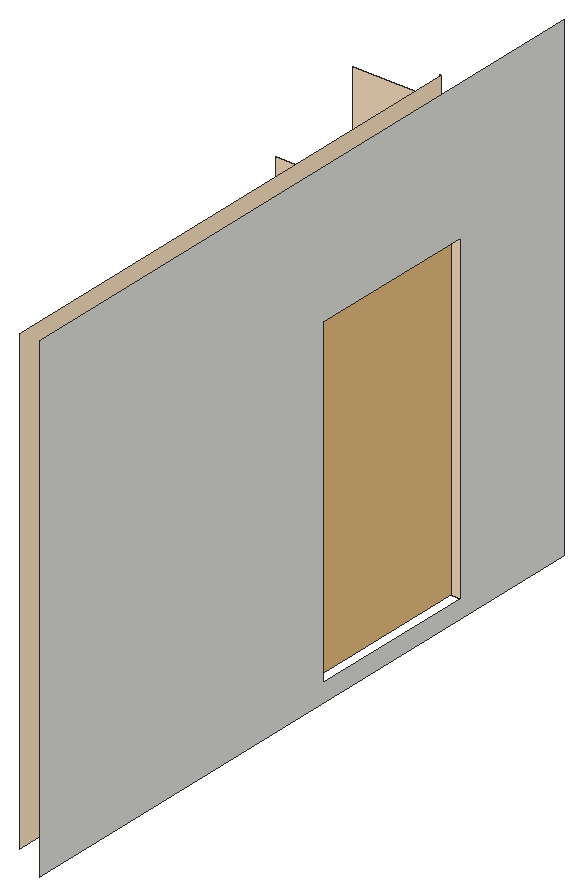
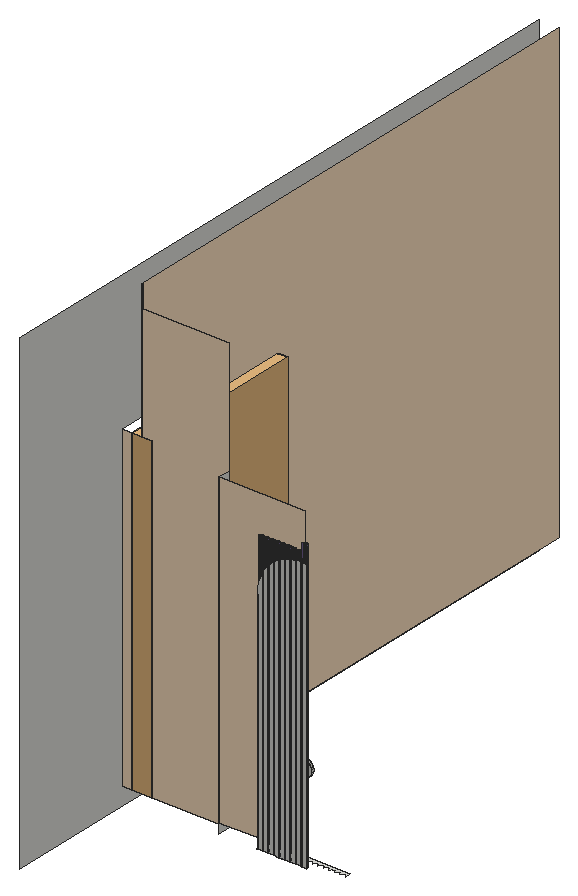
# SketchUp Ruby script. Lengths in inches.
U = 1.inch
M = Sketchup.active_model
def pt(a) = Geom::Point3d.new(a.map { |v| v * U })
def face(e, loops, mat)
  f = e.add_face(loops[0].map { |a| pt(a) })
  loops[1..].each { |l| e.add_face(l.map { |a| pt(a) }).erase! }
  f.material = f.back_material = mat if mat
  f
end
# faces: each face lists its corners as indices into pts; further lists are holes
def faces(e, pts, list, mat = nil) = list.each { |f| face(e, (f[0].is_a?(Array) ? f : [f]).map { |l| l.map { |i| pts[i] } }, mat) }
# xy, xz, yz: faces in a plane at the given z, y or x. An outline is a flat list of corners, or four numbers for a rectangle; further outlines are holes
def ring(l) = l.size == 4 ? [[l[0], l[1]], [l[2], l[1]], [l[2], l[3]], [l[0], l[3]]] : l.each_slice(2).to_a
def flat(e, list, mat, &to3) = list.each { |f| face(e, (f[0].is_a?(Array) ? f : [f]).map { |l| ring(l).map { |u, v| to3.(u, v) } }, mat) }
def xy(e, z, list, mat = nil) = flat(e, list, mat) { |x, y| [x, y, z] }
def xz(e, y, list, mat = nil) = flat(e, list, mat) { |x, z| [x, y, z] }
def yz(e, x, list, mat = nil) = flat(e, list, mat) { |y, z| [x, y, z] }
def lines(e, pts, list) = list.each { |a, b| e.add_line(pt(pts[a]), pt(pts[b])) }
# prism: a flat outline (further loops are holes) pulled along v
def prism(e, loops, v, mat = nil)
  f = face(e, loops, mat); d = Geom::Vector3d.new(v.map { |x| x * U })
  f.pushpull(f.normal.samedirection?(d) ? d.length : -d.length)
end
def box(e, o, s, mat = nil) = prism(e, [[o, [o[0] + s[0], o[1], o[2]], [o[0] + s[0], o[1] + s[1], o[2]], [o[0], o[1] + s[1], o[2]]]], [0, 0, s[2]], mat)
def at(x, y, z, deg = 0) = Geom::Transformation.translation(pt([x, y, z])) * Geom::Transformation.rotation(ORIGIN, Z_AXIS, deg.degrees)
def axes(o, x, y, z) = Geom::Transformation.new([*x, 0, *y, 0, *z, 0, *pt(o).to_a, 1])
def part(name) = M.definitions.add(name)
# library, detail: a bought-in or finely detailed component or shape, given as its bounding box
def library(name, o, s) = part(name).tap { |d| box(d.entities, o, s) }
def detail(e, o, s) = box(e.add_group.entities, o, s)
def put(e, d, t, mat = nil) = e.add_instance(d, t).tap { |i| i.material = mat if mat }
def group(e, t, mat = nil) = e.add_group.tap { |g| g.transformation = t; g.material = mat if mat }.entities
root = M.entities
M.materials.add("[0012_Bisque]").color = [255, 228, 196]
M.materials.add("[Color I01]").color = [116, 98, 147]
c1 = part("Group\#9")
xz(c1.entities,0,[[0.27,0,0.25,0.59,0.18,0.57,0.11,0.53,0.06,0.47,0.02,0.4,0,0.33,0,0.25,0.02,0.18,0.07,0.11,0.125,0.06,0.19,0.02],[0.35,0,0.42,0.02,0.49,0.07,0.54,0.125,0.58,0.19,0.6,0.27,0.59,0.35,0.57,0.42,0.53,0.49,0.47,0.54,0.4,0.58,0.33,0.6]])
xz(c1.entities,0.0625,[[0.27,0,0.35,0,0.33,0.6,0.25,0.59]])
yz(c1.entities,0,[[0,0.25,0.0625,0.33]])
p = [[0.125,0.0625,0.06],[0.19,0.0625,0.02],[0.19,0,0.02],[0.125,0,0.06],[0.27,0.0625,0],[0.27,0,0],
  [0.33,0.0625,0.6],[0.35,0.0625,0],[0.35,0,0],[0.33,0,0.6],[0.42,0.0625,0.02],[0.42,0,0.02],
  [0.25,0.0625,0.59],[0.25,0,0.59],[0.49,0.0625,0.07],[0.49,0,0.07],[0.02,0.0625,0.18],[0.07,0.0625,0.11],
  [0.07,0,0.11],[0.02,0,0.18],[0.54,0.0625,0.125],[0.54,0,0.125],[0.58,0.0625,0.19],[0.58,0,0.19],
  [0,0.0625,0.25],[0,0,0.25],[0.6,0.0625,0.27],[0.6,0,0.27],[0.02,0.0625,0.4],[0,0.0625,0.33],
  [0,0,0.33],[0.02,0,0.4],[0.59,0.0625,0.35],[0.57,0.0625,0.42],[0.57,0,0.42],[0.59,0,0.35],
  [0.06,0.0625,0.47],[0.06,0,0.47],[0.53,0.0625,0.49],[0.53,0,0.49],[0.18,0.0625,0.57],[0.11,0.0625,0.53],
  [0.11,0,0.53],[0.18,0,0.57],[0.47,0.0625,0.54],[0.4,0.0625,0.58],[0.4,0,0.58],[0.47,0,0.54]]
faces(c1.entities,p,[[0,1,2,3],[1,4,5,2],[6,7,8,9],[7,10,11,8],[4,12,13,5],[10,14,15,11],[16,17,18,19],[17,0,3,18],
  [14,20,21,15],[20,22,23,21],[24,16,19,25],[22,26,27,23],[28,29,30,31],[32,33,34,35],[26,32,35,27],[36,28,31,37],
  [33,38,39,34],[40,41,42,43],[41,36,37,42],[44,45,46,47],[38,44,47,39],[12,40,43,13],[45,6,9,46]])
c2 = library("3D DOOR",[-0.52,0,0],[35.44,5.29,86.61])
xy(root,5.5,[[188.65,140.48,188.46,140.5,188.29,140.57,188.14,140.6875,188.03,140.84,187.96,141.01,187.93,141.2,189.37,141.2,189.34,141.01,189.27,140.84,189.16,140.6875,189.01,140.57,188.84,140.5],[190.09,140.48,189.9,140.5,189.73,140.57,189.58,140.6875,189.46,140.84,189.39,141.01,189.37,141.2,190.81,141.2,190.78,141.01,190.71,140.84,190.6,140.6875,190.45,140.57,190.27,140.5],[191.52,140.48,191.34,140.5,191.17,140.57,191.02,140.6875,190.9,140.84,190.83,141.01,190.81,141.2,192.24,141.2,192.22,141.01,192.15,140.84,192.03,140.6875,191.88,140.57,191.71,140.5],[192.96,140.48,192.78,140.5,192.6,140.57,192.45,140.6875,192.34,140.84,192.27,141.01,192.24,141.2,193.68,141.2,193.66,141.01,193.58,140.84,193.47,140.6875,193.32,140.57,193.15,140.5],[194.4,140.48,194.21,140.5,194.04,140.57,193.89,140.6875,193.78,140.84,193.71,141.01,193.68,141.2,195.12,141.2,195.09,141.01,195.02,140.84,194.91,140.6875,194.76,140.57,194.59,140.5],
  [195.84,140.48,195.65,140.5,195.48,140.57,195.33,140.6875,195.21,140.84,195.14,141.01,195.12,141.2,196.56,141.2,196.53,141.01,196.46,140.84,196.35,140.6875,196.2,140.57,196.02,140.5],[197.27,140.48,197.09,140.5,196.92,140.57,196.77,140.6875,196.65,140.84,196.58,141.01,196.56,141.2,197.99,141.2,197.97,141.01,197.9,140.84,197.78,140.6875,197.63,140.57,197.46,140.5],[198.71,140.48,198.53,140.5,198.35,140.57,198.2,140.6875,198.09,140.84,198.02,141.01,197.99,141.2,199.35,141.2,199.35,140.87,199.33,140.84,199.22,140.6875,199.07,140.57,198.9,140.5],[186.96,140.52,186.78,140.55,186.62,140.61,186.48,140.72,186.375,140.86,186.31,141.02,186.29,141.2,187.63,141.2,187.61,141.02,187.54,140.86,187.43,140.72,187.29,140.61,187.13,140.55],[199.35,140.87,199.41,141.01,199.43,141.2,199.35,141.2]])
xy(root,7.1875,[[176.22,139.88,199.35,139.88,199.35,140.87,199.33,140.84,199.22,140.6875,199.07,140.57,198.9,140.5,198.71,140.48,198.53,140.5,198.35,140.57,198.2,140.6875,198.09,140.84,198.02,141.01,197.99,141.2,197.97,141.01,197.9,140.84,197.78,140.6875,197.63,140.57,197.46,140.5,197.27,140.48,197.09,140.5,196.92,140.57,196.77,140.6875,196.65,140.84,196.58,141.01,196.56,141.2,196.53,141.01,196.46,140.84,196.35,140.6875,196.2,140.57,196.02,140.5,195.84,140.48,195.65,140.5,195.48,140.57,195.33,140.6875,195.21,140.84,195.14,141.01,195.12,141.2,195.09,141.01,195.02,140.84,194.91,140.6875,194.76,140.57,194.59,140.5,194.4,140.48,194.21,140.5,194.04,140.57,193.89,140.6875,193.78,140.84,193.71,141.01,193.68,141.2,193.66,141.01,193.58,140.84,193.47,140.6875,193.32,140.57,193.15,140.5,192.96,140.48,192.78,140.5,192.6,140.57,192.45,140.6875,192.34,140.84,192.27,141.01,192.24,141.2,192.22,141.01,192.15,140.84,192.03,140.6875,191.88,140.57,191.71,140.5,191.52,140.48,191.34,140.5,191.17,140.57,191.02,140.6875,190.9,140.84,190.83,141.01,190.81,141.2,190.78,141.01,190.71,140.84,190.6,140.6875,190.45,140.57,190.27,140.5,190.09,140.48,189.9,140.5,189.73,140.57,189.58,140.6875,189.46,140.84,189.39,141.01,189.37,141.2,189.34,141.01,189.27,140.84,189.16,140.6875,189.01,140.57,188.84,140.5,188.65,140.48,188.46,140.5,188.29,140.57,188.14,140.6875,188.03,140.84,187.96,141.01,187.93,141.2,187.63,141.2,187.61,141.02,187.54,140.86,187.43,140.72,187.29,140.61,187.13,140.55,186.96,140.52,186.78,140.55,186.62,140.61,186.48,140.72,186.375,140.86,186.31,141.02,186.29,141.2,186.26,141.01,186.19,140.84,186.08,140.6875,185.93,140.57,185.75,140.5,185.57,140.48,185.38,140.5,185.21,140.57,185.06,140.6875,184.94,140.84,184.875,141.01,184.85,141.2,184.82,141.01,184.75,140.84,184.64,140.6875,184.49,140.57,184.32,140.5,184.13,140.48,183.94,140.5,183.77,140.57,183.62,140.6875,183.51,140.84,183.4375,141.01,183.41,141.2,183.39,141.01,183.31,140.84,183.2,140.6875,183.05,140.57,182.88,140.5,182.69,140.48,182.51,140.5,182.33,140.57,182.18,140.6875,182.07,140.84,182,141.01,181.97,141.2,181.95,141.01,181.88,140.84,181.76,140.6875,181.61,140.57,181.44,140.5,181.25,140.48,181.07,140.5,180.9,140.57,180.75,140.6875,180.63,140.84,180.5625,141.01,180.54,141.2,180.51,141.01,180.44,140.84,180.33,140.6875,180.18,140.57,180,140.5,179.82,140.48,179.63,140.5,179.46,140.57,179.31,140.6875,179.19,140.84,179.125,141.01,179.1,141.2,179.07,141.01,179,140.84,178.89,140.6875,178.74,140.57,178.57,140.5,178.38,140.48,178.19,140.5,178.02,140.57,177.87,140.6875,177.76,140.84,177.6875,141.01,177.66,141.2,177.64,141.01,177.56,140.84,177.45,140.6875,177.3,140.57,177.13,140.5,176.94,140.48,176.76,140.5,176.58,140.57,176.43,140.6875,176.32,140.84,176.25,141.01,176.22,141.2]])
xz(root,92.18,[[233.26,4.6875,238.375,88.6875]])
xz(root,136.82,[[210.45,4.6875,238.375,4.6875,238.375,88.6875,233.26,88.6875,233.26,124.6875,232.96,124.6875,232.96,118.75,210.45,118.75]],"[0012_Bisque]")
xz(root,139.88,[[199.35,7.1875,210.45,7.1875,210.45,88.4375,187.93,88.4375,187.93,76.97,187.9375,76.97,188.24,76.96,188.55,76.95,189.15,76.89,189.46,76.85,190.06,76.75,190.36,76.68,190.65,76.61,190.95,76.53,191.53,76.35,191.82,76.25,192.1,76.14,192.38,76.02,192.66,75.89,192.9375,75.76,193.21,75.62,193.48,75.47,193.74,75.32,194,75.16,194.26,74.99,194.51,74.82,194.75,74.64,195.23,74.26,195.46,74.06,195.6875,73.85,195.91,73.64,196.33,73.2,196.73,72.74,196.92,72.5,197.1,72.26,197.28,72.01,197.45,71.75,197.62,71.5,197.77,71.24,198.07,70.7,198.2,70.43,198.33,70.15,198.57,69.59,198.77,69.01,198.95,68.43,199.09,67.83,199.15,67.53,199.25,66.93,199.28,66.63,199.3125,66.32,199.33,66.02,199.34,65.71,199.35,65.41]],"[0012_Bisque]")
xz(root,141.2,[[186.29,5.5,187.63,5.5,187.63,76.95,187.33,76.96,187.03,76.95,186.43,76.89,186.29,76.875],[187.93,5.5,189.37,5.5,189.37,76.86,189.15,76.89,188.55,76.95,188.24,76.96,187.9375,76.97,187.93,76.97],[189.37,5.5,190.81,5.5,190.81,76.57,190.65,76.61,190.36,76.68,190.06,76.75,189.46,76.85,189.37,76.86],[190.81,5.5,192.24,5.5,192.24,76.08,192.1,76.14,191.82,76.25,191.53,76.35,190.95,76.53,190.81,76.57],[192.24,5.5,193.68,5.5,193.68,75.36,193.48,75.47,193.21,75.62,192.9375,75.76,192.66,75.89,192.38,76.02,192.24,76.08],
  [193.68,5.5,195.12,5.5,195.12,74.35,194.99,74.45,194.75,74.64,194.51,74.82,194.26,74.99,194,75.16,193.74,75.32,193.68,75.36],[195.12,5.5,196.56,5.5,196.56,72.94,196.53,72.97,196.33,73.2,195.91,73.64,195.6875,73.85,195.46,74.06,195.23,74.26,195.12,74.35],[196.56,5.5,197.99,5.5,197.99,70.84,197.92,70.97,197.77,71.24,197.62,71.5,197.45,71.75,197.28,72.01,197.1,72.26,196.92,72.5,196.73,72.74,196.56,72.94],[197.99,5.5,197.99,70.84,198.07,70.7,198.2,70.43,198.33,70.15,198.57,69.59,198.77,69.01,198.95,68.43,199.09,67.83,199.15,67.53,199.25,66.93,199.28,66.63,199.3125,66.32,199.33,66.02,199.34,65.71,199.35,65.41,199.35,5.5],[187.63,7.1875,187.93,7.1875,187.93,76.97,187.63,76.95]])
yz(root,199.35,[[140.87,5.5,141.2,65.41],[139.88,7.1875,140.87,65.41]])
yz(root,210.45,[[136.82,4.6875,139.88,88.4375]])
yz(root,233.26,[[0,4.6875,0,124.6875,136.82,124.6875,136.82,88.6875,92.18,88.6875,92.18,4.6875]],"[0012_Bisque]")
yz(root,238.375,[[[0,0,170.3125,124.6875],[92.18,4.6875,136.82,88.6875]]])
p = [[186.62,140.61,5.5],[186.78,140.55,5.5],[186.78,140.55,7.1875],[186.62,140.61,7.1875],[186.96,140.52,5.5],[186.96,140.52,7.1875],
  [187.13,140.55,5.5],[187.13,140.55,7.1875],[187.29,140.61,5.5],[187.29,140.61,7.1875],[188.29,140.57,5.5],[188.46,140.5,5.5],
  [188.46,140.5,7.1875],[188.29,140.57,7.1875],[188.65,140.48,5.5],[188.65,140.48,7.1875],[188.84,140.5,5.5],[188.84,140.5,7.1875],
  [189.01,140.57,5.5],[189.01,140.57,7.1875],[189.73,140.57,5.5],[189.9,140.5,5.5],[189.9,140.5,7.1875],[189.73,140.57,7.1875],
  [190.09,140.48,5.5],[190.09,140.48,7.1875],[190.27,140.5,5.5],[190.27,140.5,7.1875],[190.45,140.57,5.5],[190.45,140.57,7.1875],
  [191.17,140.57,5.5],[191.34,140.5,5.5],[191.34,140.5,7.1875],[191.17,140.57,7.1875],[191.52,140.48,5.5],[191.52,140.48,7.1875],
  [191.71,140.5,5.5],[191.71,140.5,7.1875],[191.88,140.57,5.5],[191.88,140.57,7.1875],[192.6,140.57,5.5],[192.78,140.5,5.5],
  [192.78,140.5,7.1875],[192.6,140.57,7.1875],[192.96,140.48,5.5],[192.96,140.48,7.1875],[193.15,140.5,5.5],[193.15,140.5,7.1875],
  [193.32,140.57,5.5],[193.32,140.57,7.1875],[194.04,140.57,5.5],[194.21,140.5,5.5],[194.21,140.5,7.1875],[194.04,140.57,7.1875],
  [194.4,140.48,5.5],[194.4,140.48,7.1875],[194.59,140.5,5.5],[194.59,140.5,7.1875],[194.76,140.57,5.5],[194.76,140.57,7.1875],
  [195.48,140.57,5.5],[195.65,140.5,5.5],[195.65,140.5,7.1875],[195.48,140.57,7.1875],[195.84,140.48,5.5],[195.84,140.48,7.1875],
  [196.02,140.5,5.5],[196.02,140.5,7.1875],[196.2,140.57,5.5],[196.2,140.57,7.1875],[196.92,140.57,5.5],[197.09,140.5,5.5],
  [197.09,140.5,7.1875],[196.92,140.57,7.1875],[197.27,140.48,5.5],[197.27,140.48,7.1875],[197.46,140.5,5.5],[197.46,140.5,7.1875],
  [197.63,140.57,5.5],[197.63,140.57,7.1875],[198.35,140.57,5.5],[198.53,140.5,5.5],[198.53,140.5,7.1875],[198.35,140.57,7.1875],
  [198.71,140.48,5.5],[198.71,140.48,7.1875],[198.9,140.5,5.5],[198.9,140.5,7.1875],[199.07,140.57,5.5],[199.07,140.57,7.1875],
  [186.48,140.72,5.5],[186.48,140.72,7.1875],[187.43,140.72,5.5],[187.43,140.72,7.1875],[188.14,140.6875,5.5],[188.14,140.6875,7.1875],
  [189.16,140.6875,5.5],[189.16,140.6875,7.1875],[189.58,140.6875,5.5],[189.58,140.6875,7.1875],[190.6,140.6875,5.5],[190.6,140.6875,7.1875],
  [191.02,140.6875,5.5],[191.02,140.6875,7.1875],[192.03,140.6875,5.5],[192.03,140.6875,7.1875],[192.45,140.6875,5.5],[192.45,140.6875,7.1875],
  [193.47,140.6875,5.5],[193.47,140.6875,7.1875],[193.89,140.6875,5.5],[193.89,140.6875,7.1875],[194.91,140.6875,5.5],[194.91,140.6875,7.1875],
  [195.33,140.6875,5.5],[195.33,140.6875,7.1875],[196.35,140.6875,5.5],[196.35,140.6875,7.1875],[196.77,140.6875,5.5],[196.77,140.6875,7.1875],
  [197.78,140.6875,5.5],[197.78,140.6875,7.1875],[198.2,140.6875,7.1875],[198.2,140.6875,5.5],[199.22,140.6875,5.5],[199.22,140.6875,7.1875],
  [186.375,140.86,5.5],[186.375,140.86,7.1875],[187.54,140.86,5.5],[187.54,140.86,7.1875],[188.03,140.84,5.5],[188.03,140.84,7.1875],
  [189.27,140.84,5.5],[189.27,140.84,7.1875],[189.46,140.84,5.5],[189.46,140.84,7.1875],[190.71,140.84,5.5],[190.71,140.84,7.1875],
  [190.9,140.84,5.5],[190.9,140.84,7.1875],[192.15,140.84,5.5],[192.15,140.84,7.1875],[192.34,140.84,5.5],[192.34,140.84,7.1875],
  [193.58,140.84,5.5],[193.58,140.84,7.1875],[193.78,140.84,5.5],[193.78,140.84,7.1875],[195.02,140.84,5.5],[195.02,140.84,7.1875],
  [195.21,140.84,5.5],[195.21,140.84,7.1875],[196.46,140.84,5.5],[196.46,140.84,7.1875],[196.65,140.84,5.5],[196.65,140.84,7.1875],
  [197.9,140.84,5.5],[197.9,140.84,7.1875],[198.09,140.84,7.1875],[198.09,140.84,5.5],[199.33,140.84,5.5],[199.33,140.84,7.1875],
  [187.96,141.01,5.5],[187.96,141.01,7.1875],[189.34,141.01,5.5],[189.34,141.01,7.1875],[189.39,141.01,5.5],[189.39,141.01,7.1875],
  [190.78,141.01,5.5],[190.78,141.01,7.1875],[190.83,141.01,5.5],[190.83,141.01,7.1875],[192.22,141.01,5.5],[192.22,141.01,7.1875],
  [192.27,141.01,5.5],[192.27,141.01,7.1875],[193.66,141.01,5.5],[193.66,141.01,7.1875],[193.71,141.01,5.5],[193.71,141.01,7.1875],
  [195.09,141.01,5.5],[195.09,141.01,7.1875],[195.14,141.01,5.5],[195.14,141.01,7.1875],[196.53,141.01,5.5],[196.53,141.01,7.1875],
  [196.58,141.01,5.5],[196.58,141.01,7.1875],[197.97,141.01,5.5],[197.97,141.01,7.1875],[198.02,141.01,5.5],[198.02,141.01,7.1875],
  [199.35,140.87,5.5],[199.35,140.87,7.1875],[186.31,141.02,5.5],[186.31,141.02,7.1875],[187.61,141.02,5.5],[187.61,141.02,7.1875],
  [186.29,141.2,5.5],[186.29,141.2,7.1875],[187.63,141.2,5.5],[187.63,141.2,7.1875],[187.93,141.2,5.5],[187.93,141.2,7.1875],
  [189.37,141.2,5.5],[189.37,141.2,7.1875],[190.81,141.2,5.5],[190.81,141.2,7.1875],[192.24,141.2,5.5],[192.24,141.2,7.1875],
  [193.68,141.2,5.5],[193.68,141.2,7.1875],[195.12,141.2,5.5],[195.12,141.2,7.1875],[196.56,141.2,5.5],[196.56,141.2,7.1875],
  [197.99,141.2,5.5],[197.99,141.2,7.1875],[186.62,140.61,81.5],[186.78,140.55,81.5],[186.96,140.52,81.5],[187.13,140.55,81.5],
  [187.29,140.61,81.5],[188.29,140.57,79.3125],[188.46,140.5,79.3125],[188.65,140.48,79.3125],[188.84,140.5,79.3125],[189.01,140.57,79.3125],
  [189.73,140.57,79.3125],[189.9,140.5,79.3125],[190.09,140.48,79.3125],[190.27,140.5,79.3125],[190.45,140.57,79.3125],[191.17,140.57,79.3125],
  [191.34,140.5,79.3125],[191.52,140.48,79.3125],[191.71,140.5,79.3125],[191.88,140.57,79.3125],[192.6,140.57,79.3125],[192.78,140.5,79.3125],
  [192.96,140.48,79.3125],[193.15,140.5,79.3125],[193.32,140.57,79.3125],[194.04,140.57,79.3125],[194.21,140.5,79.3125],[194.4,140.48,79.3125],
  [194.59,140.5,79.3125],[194.76,140.57,79.3125],[195.48,140.57,79.3125],[195.65,140.5,79.3125],[195.84,140.48,79.3125],[196.02,140.5,79.3125],
  [196.2,140.57,79.3125],[196.92,140.57,79.3125],[197.09,140.5,79.3125],[197.27,140.48,79.3125],[197.46,140.5,79.3125],[197.63,140.57,79.3125],
  [198.35,140.57,79.3125],[198.53,140.5,79.3125],[198.71,140.48,79.3125],[198.9,140.5,79.3125],[199.07,140.57,79.3125],[186.48,140.72,81.5],
  [187.43,140.72,81.5],[188.14,140.6875,79.3125],[189.16,140.6875,79.3125],[189.58,140.6875,79.3125],[190.6,140.6875,79.3125],[191.02,140.6875,79.3125],
  [192.03,140.6875,79.3125],[192.45,140.6875,79.3125],[193.47,140.6875,79.3125],[193.89,140.6875,79.3125],[194.91,140.6875,79.3125],[195.33,140.6875,79.3125],
  [196.35,140.6875,79.3125],[196.77,140.6875,79.3125],[197.78,140.6875,79.3125],[198.2,140.6875,70.43],[198.2,140.6875,79.3125],[199.22,140.6875,79.3125],
  [186.375,140.86,81.5],[187.54,140.86,81.5],[188.03,140.84,79.3125],[189.27,140.84,79.3125],[189.46,140.84,79.3125],[190.71,140.84,79.3125],
  [190.9,140.84,79.3125],[192.15,140.84,79.3125],[192.34,140.84,79.3125],[193.58,140.84,79.3125],[193.78,140.84,79.3125],[195.02,140.84,79.3125],
  [195.21,140.84,79.3125],[196.46,140.84,79.3125],[196.65,140.84,79.3125],[197.9,140.84,79.3125],[198.09,140.84,79.3125],[199.33,140.84,79.3125],
  [187.96,141.01,79.3125],[189.34,141.01,79.3125],[189.39,141.01,79.3125],[190.78,141.01,79.3125],[190.83,141.01,79.3125],[192.22,141.01,79.3125],
  [192.27,141.01,79.3125],[193.66,141.01,79.3125],[193.71,141.01,79.3125],[195.09,141.01,79.3125],[195.14,141.01,79.3125],[196.53,141.01,79.3125],
  [196.58,141.01,79.3125],[197.97,141.01,79.3125],[198.02,141.01,79.3125],[199.35,140.87,65.41],[199.35,140.87,79.3125],[186.31,141.02,81.5],
  [187.61,141.02,81.5],[186.29,141.2,76.875],[186.29,141.2,81.5],[187.63,141.2,76.95],[187.63,141.2,81.5],[187.93,141.2,76.95],
  [187.93,141.2,79.3125],[187.93,141.2,76.97],[189.37,141.2,76.86],[189.37,141.2,79.3125],[190.81,141.2,76.57],[190.81,141.2,79.3125],
  [192.24,141.2,76.08],[192.24,141.2,79.3125],[193.68,141.2,75.36],[193.68,141.2,79.3125],[195.12,141.2,74.35],[195.12,141.2,79.3125],
  [196.56,141.2,72.94],[196.56,141.2,79.3125],[197.99,141.2,70.84],[197.99,141.2,79.3125]]
faces(root,p,[[0,1,2,3],[1,4,5,2],[4,6,7,5],[6,8,9,7],[10,11,12,13],[11,14,15,12],[14,16,17,15],[16,18,19,17],
  [20,21,22,23],[21,24,25,22],[24,26,27,25],[26,28,29,27],[30,31,32,33],[31,34,35,32],[34,36,37,35],[36,38,39,37],
  [40,41,42,43],[41,44,45,42],[44,46,47,45],[46,48,49,47],[50,51,52,53],[51,54,55,52],[54,56,57,55],[56,58,59,57],
  [60,61,62,63],[61,64,65,62],[64,66,67,65],[66,68,69,67],[70,71,72,73],[71,74,75,72],[74,76,77,75],[76,78,79,77],
  [80,81,82,83],[81,84,85,82],[84,86,87,85],[86,88,89,87],[90,0,3,91],[8,92,93,9],[94,10,13,95],[18,96,97,19],
  [98,20,23,99],[28,100,101,29],[102,30,33,103],[38,104,105,39],[106,40,43,107],[48,108,109,49],[110,50,53,111],[58,112,113,59],
  [114,60,63,115],[68,116,117,69],[118,70,73,119],[78,120,121,79],[80,83,122,123],[88,124,125,89],[126,90,91,127],[92,128,129,93],
  [130,94,95,131],[96,132,133,97],[134,98,99,135],[100,136,137,101],[138,102,103,139],[104,140,141,105],[142,106,107,143],[108,144,145,109],
  [146,110,111,147],[112,148,149,113],[150,114,115,151],[116,152,153,117],[154,118,119,155],[120,156,157,121],[123,122,158,159],[124,160,161,125],
  [162,130,131,163],[132,164,165,133],[166,134,135,167],[136,168,169,137],[170,138,139,171],[140,172,173,141],[174,142,143,175],[144,176,177,145],
  [178,146,147,179],[148,180,181,149],[182,150,151,183],[152,184,185,153],[186,154,155,187],[156,188,189,157],[190,159,158,191],[160,192,193,161],
  [194,126,127,195],[128,196,197,129],[198,194,195,199],[196,200,201,197],[202,162,163,203],[164,204,205,165],[204,166,167,205],[168,206,207,169],
  [206,170,171,207],[172,208,209,173],[208,174,175,209],[176,210,211,177],[210,178,179,211],[180,212,213,181],[212,182,183,213],[184,214,215,185],
  [214,186,187,215],[188,216,217,189],[216,190,191,217]])
faces(root,p,[[218,3,2,219],[219,2,5,220],[220,5,7,221],[221,7,9,222],[223,13,12,224],[224,12,15,225],[225,15,17,226],[226,17,19,227],
  [228,23,22,229],[229,22,25,230],[230,25,27,231],[231,27,29,232],[233,33,32,234],[234,32,35,235],[235,35,37,236],[236,37,39,237],
  [238,43,42,239],[239,42,45,240],[240,45,47,241],[241,47,49,242],[243,53,52,244],[244,52,55,245],[245,55,57,246],[246,57,59,247],
  [248,63,62,249],[249,62,65,250],[250,65,67,251],[251,67,69,252],[253,73,72,254],[254,72,75,255],[255,75,77,256],[256,77,79,257],
  [258,83,82,259],[259,82,85,260],[260,85,87,261],[261,87,89,262],[263,91,3,218],[222,9,93,264],[265,95,13,223],[227,19,97,266],
  [267,99,23,228],[232,29,101,268],[269,103,33,233],[237,39,105,270],[271,107,43,238],[242,49,109,272],[273,111,53,243],[247,59,113,274],
  [275,115,63,248],[252,69,117,276],[277,119,73,253],[257,79,121,278],[279,122,83,258,280],[262,89,125,281],[282,127,91,263],[264,93,129,283],
  [284,131,95,265],[266,97,133,285],[286,135,99,267],[268,101,137,287],[288,139,103,269],[270,105,141,289],[290,143,107,271],[272,109,145,291],
  [292,147,111,273],[274,113,149,293],[294,151,115,275],[276,117,153,295],[296,155,119,277],[278,121,157,297],[298,158,122,279,280],[281,125,161,299],
  [300,163,131,284],[285,133,165,301],[302,167,135,286],[287,137,169,303],[304,171,139,288],[289,141,173,305],[306,175,143,290],[291,145,177,307],
  [308,179,147,292],[293,149,181,309],[310,183,151,294],[295,153,185,311],[312,187,155,296],[297,157,189,313],[314,191,158,298],[299,161,193,315,316],
  [317,195,127,282],[283,129,197,318],[319,199,195,317,320],[318,197,201,321,322],[323,203,163,300,324,325],[301,165,205,326,327],[326,205,167,302,327],[303,169,207,328,329],
  [328,207,171,304,329],[305,173,209,330,331],[330,209,175,306,331],[307,177,211,332,333],[332,211,179,308,333],[309,181,213,334,335],[334,213,183,310,335],[311,185,215,336,337],
  [336,215,187,312,337],[313,189,217,338,339],[338,217,191,314,339]],"[Color I01]")
put(root,c1,axes([185.43,140.2,26.13],[7.7976,0,0],[0,7.7976,0],[0,0,7.7976]))
put(root,c2,axes([230.51,136.17,4.6875],[0,-1.26,0],[1,0,0],[0,0,0.96982]))
